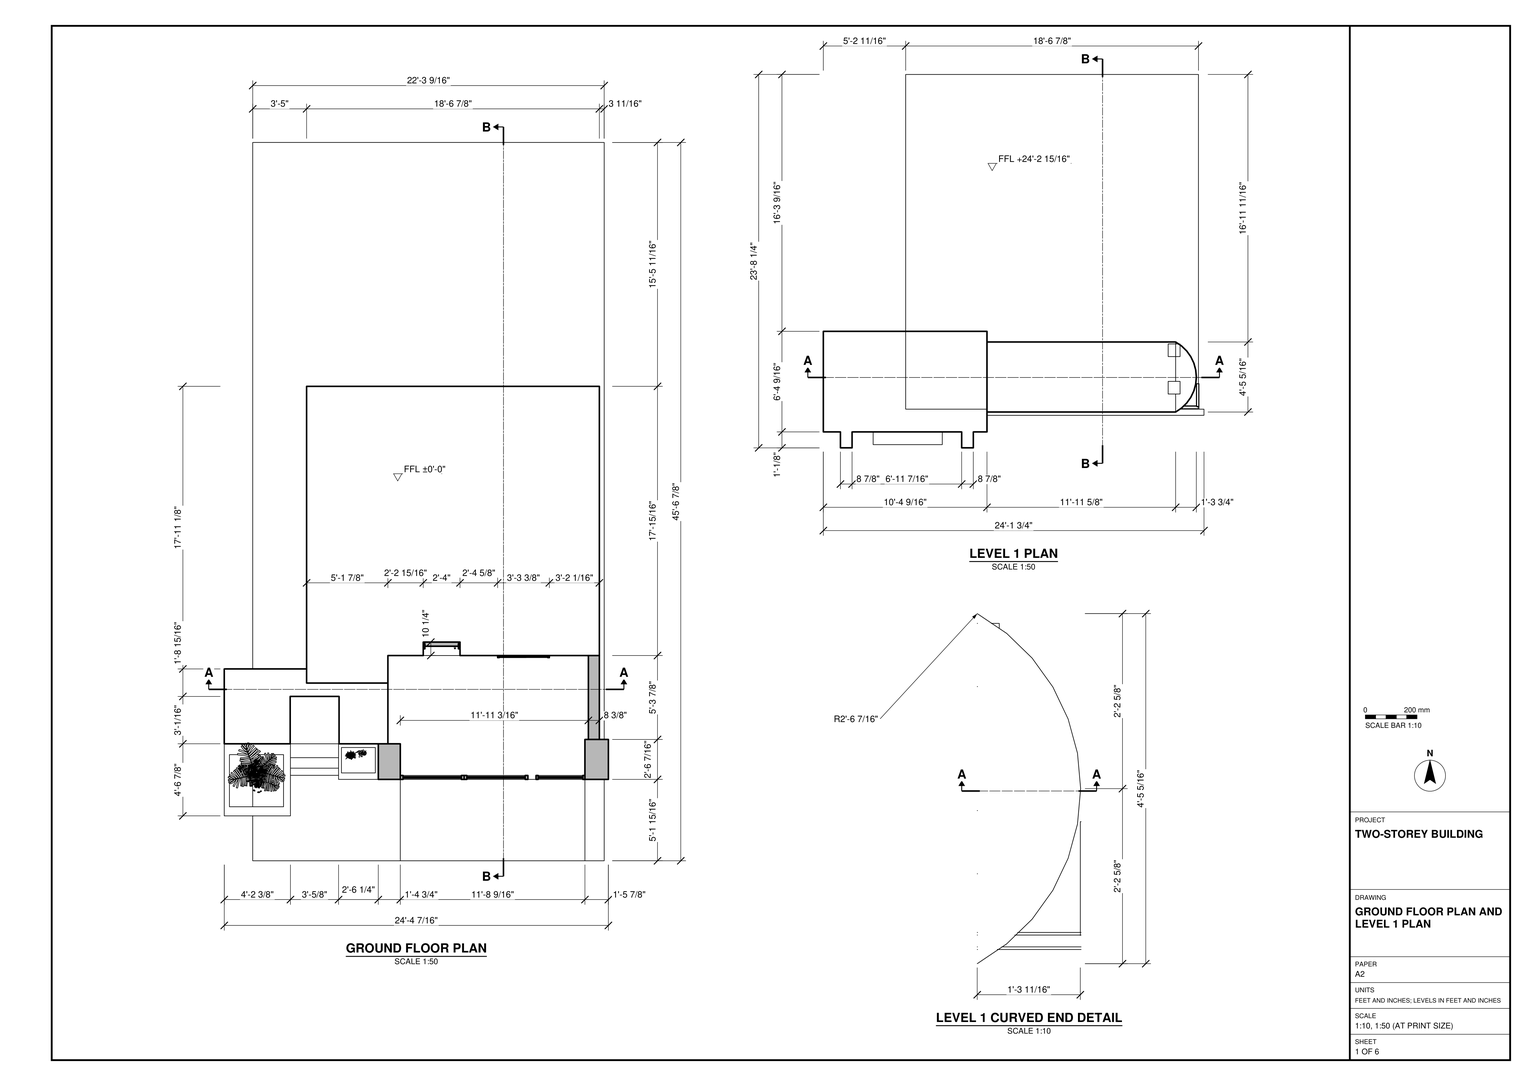
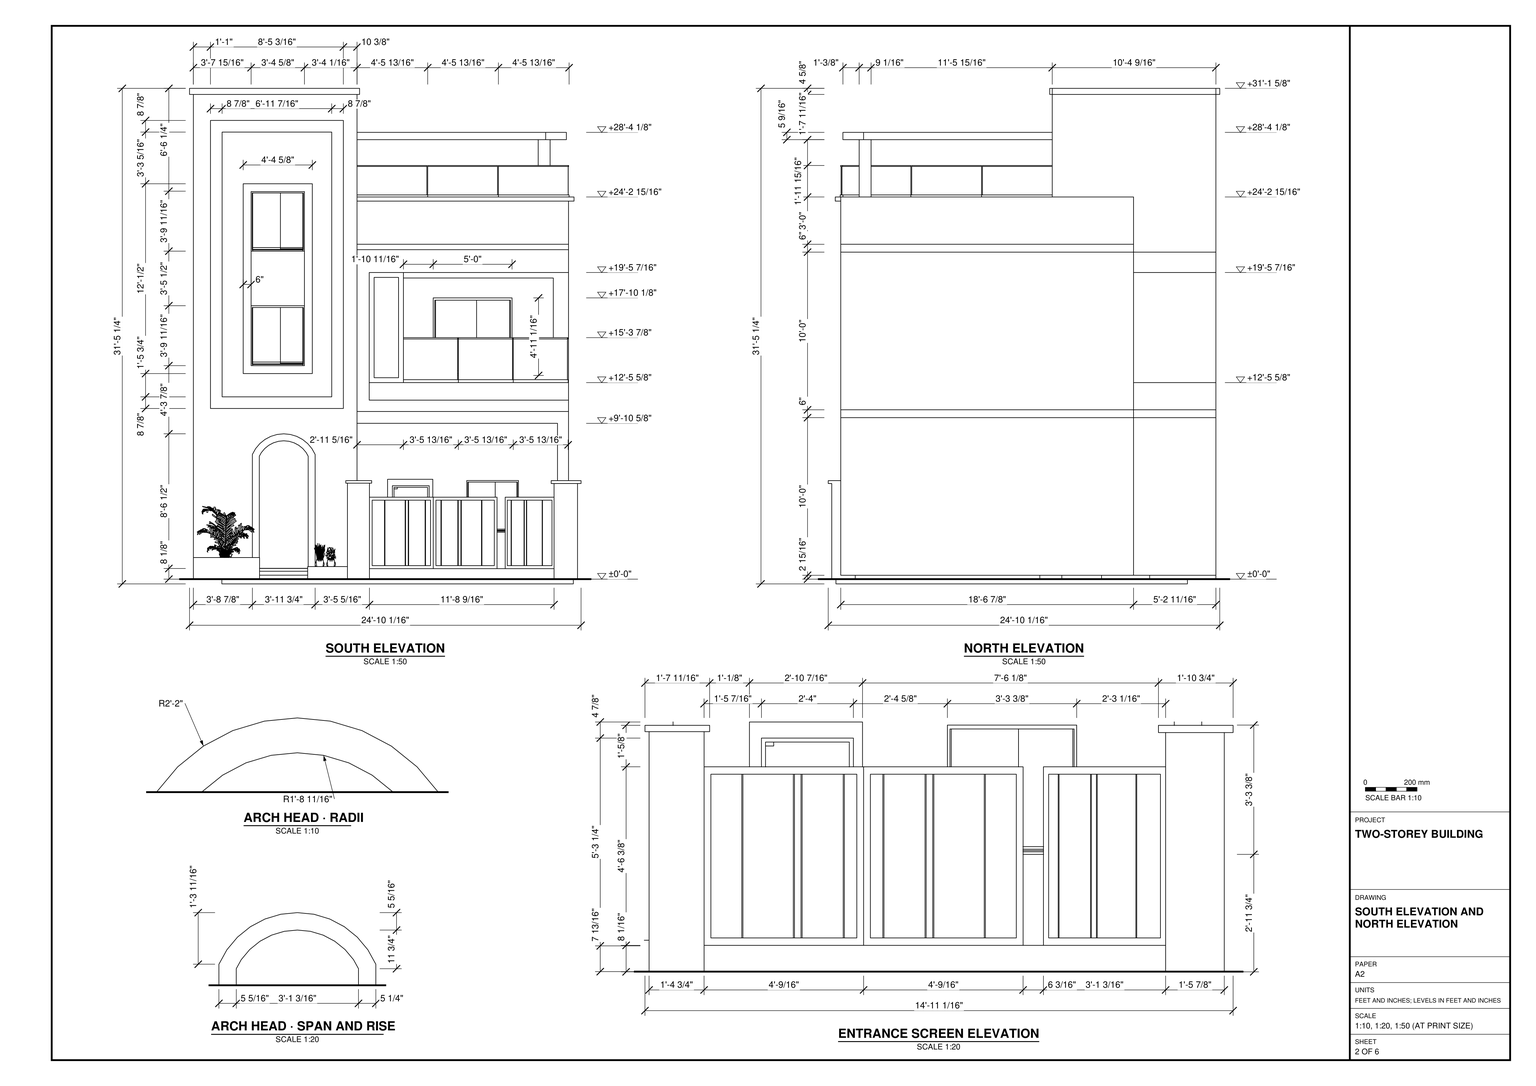
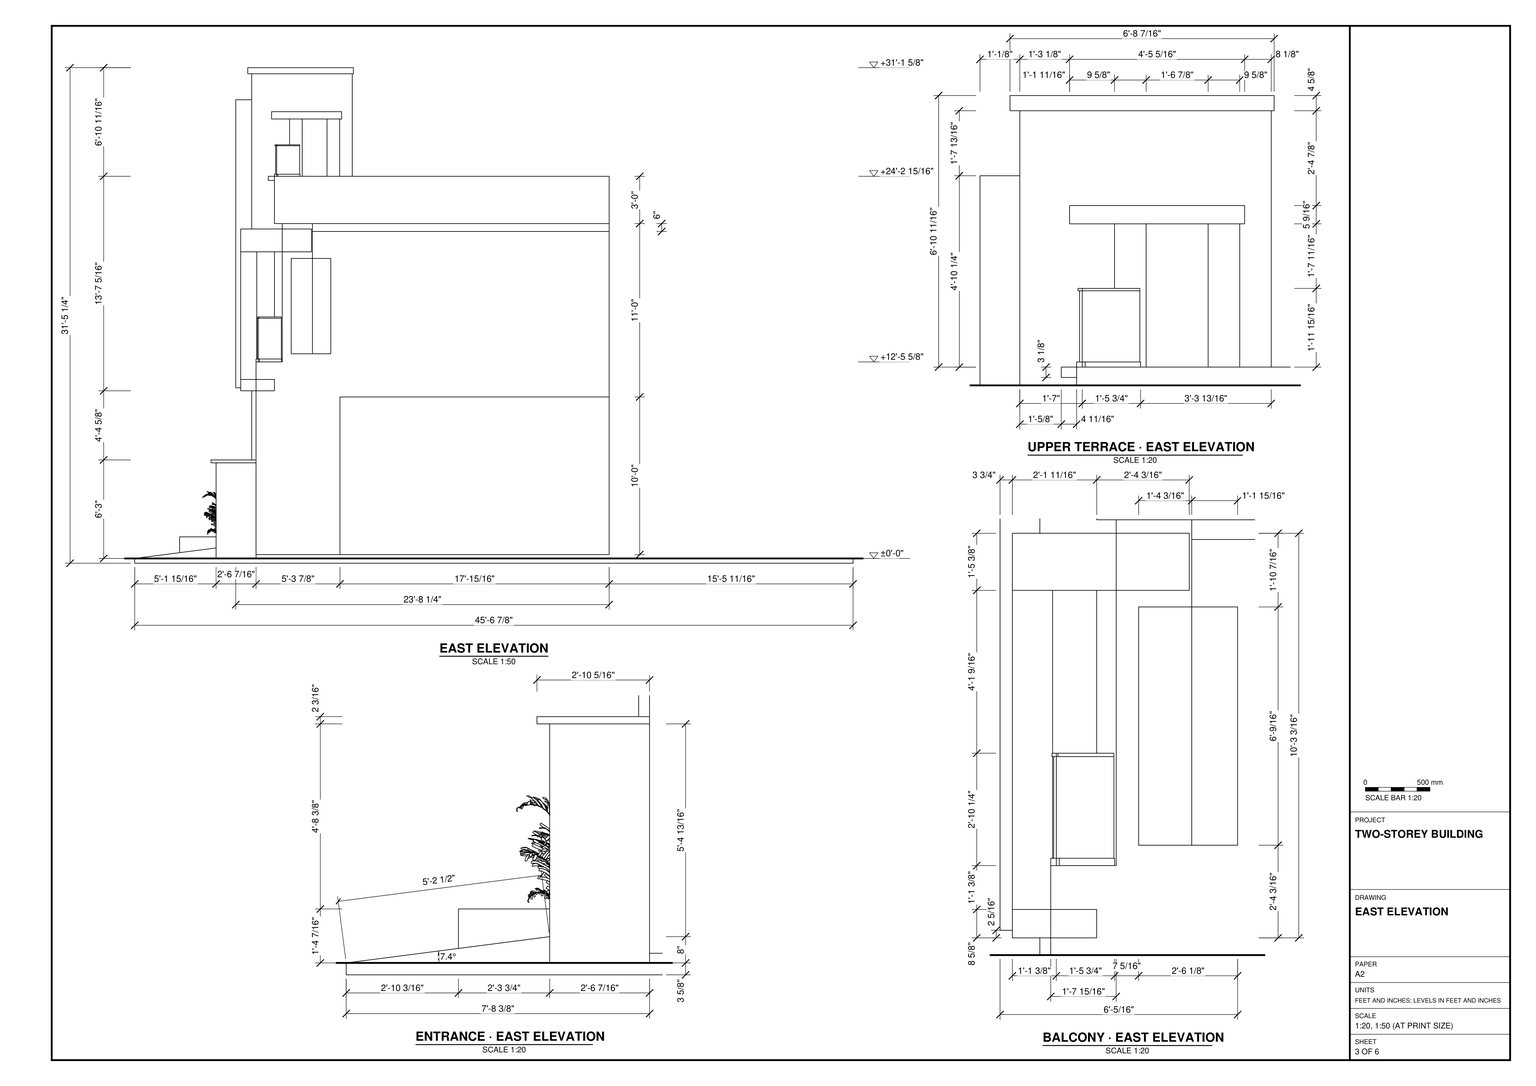
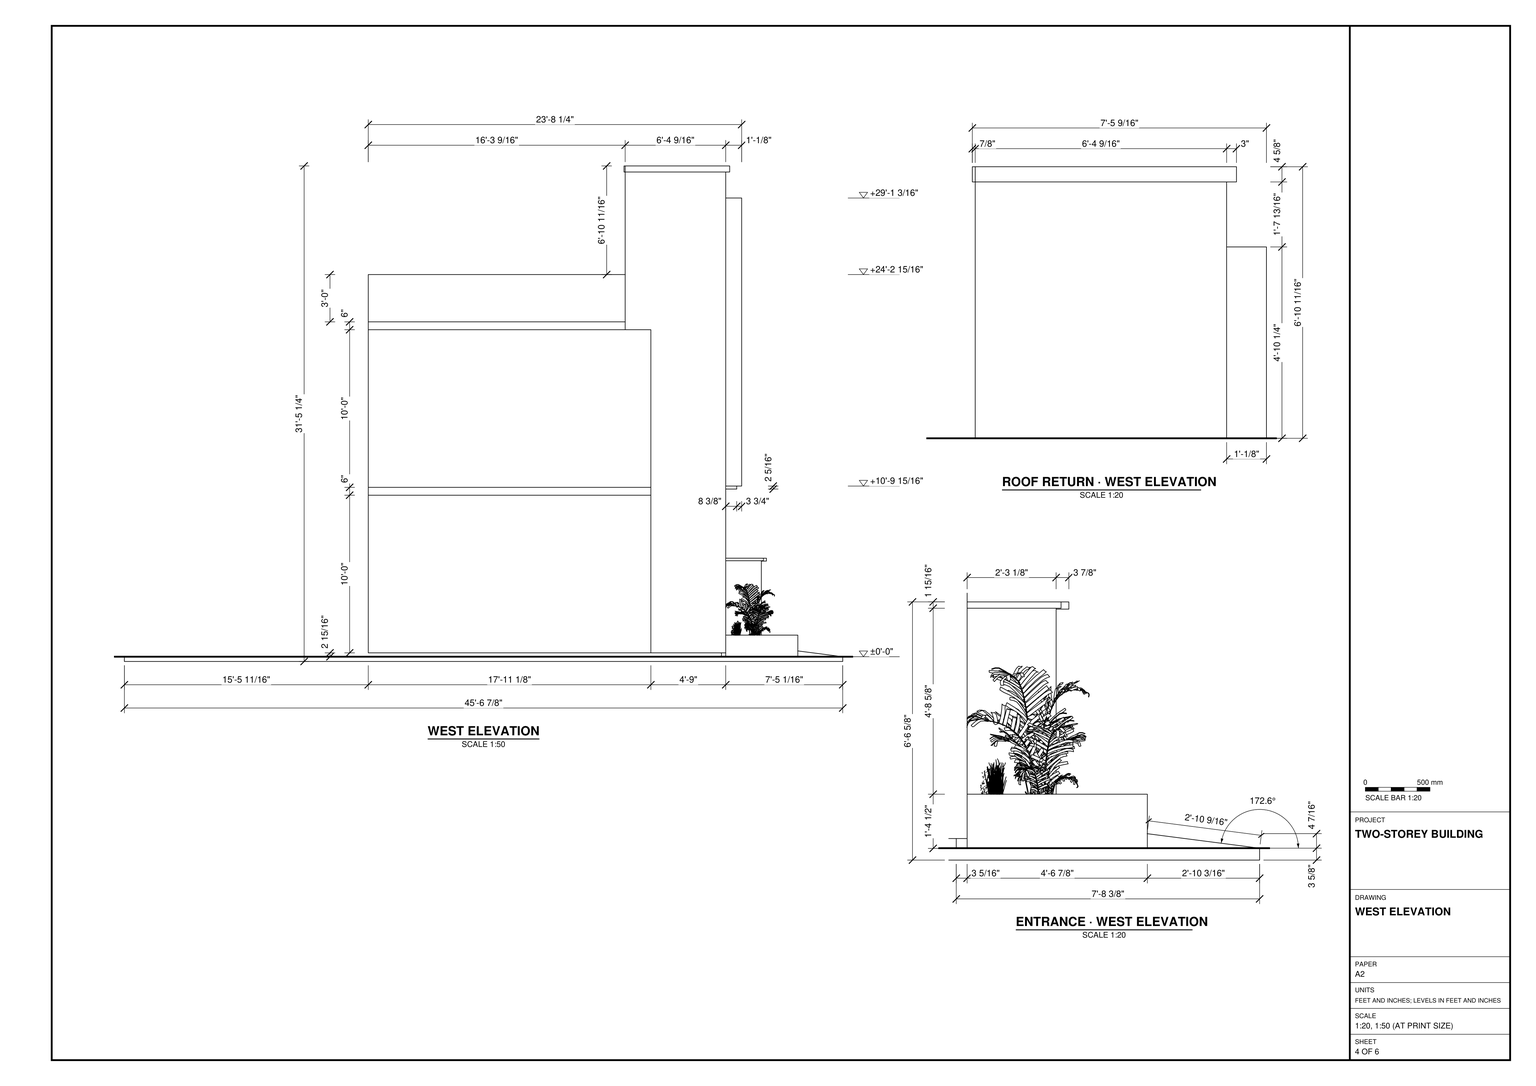
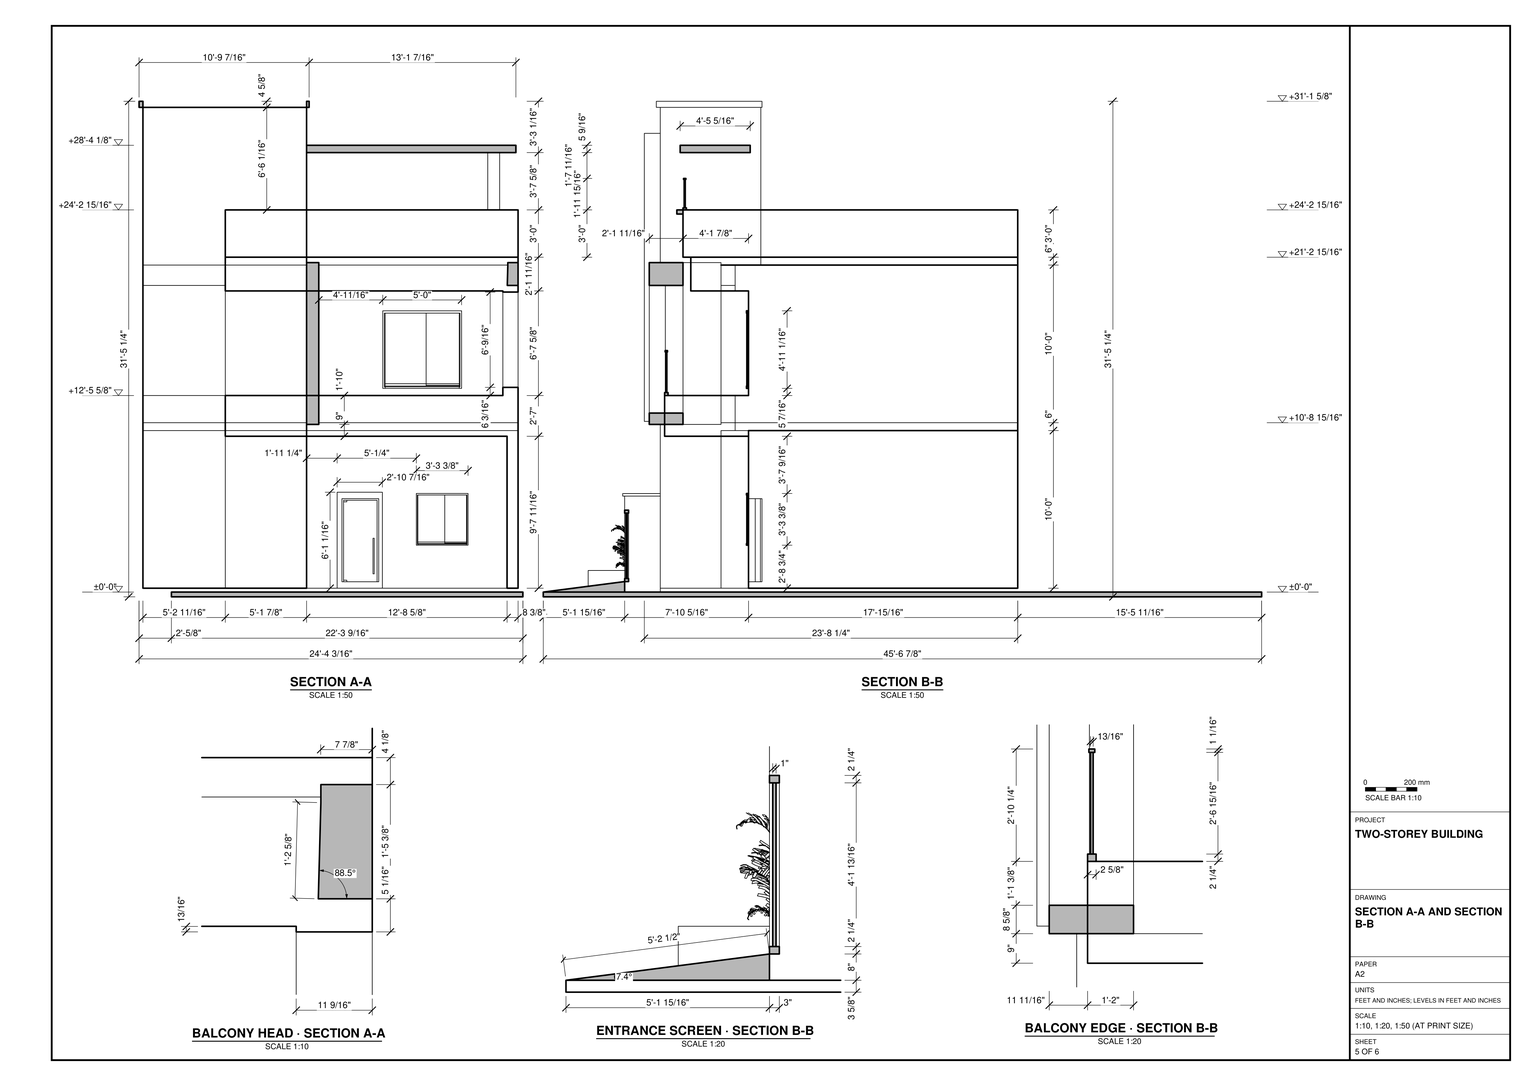
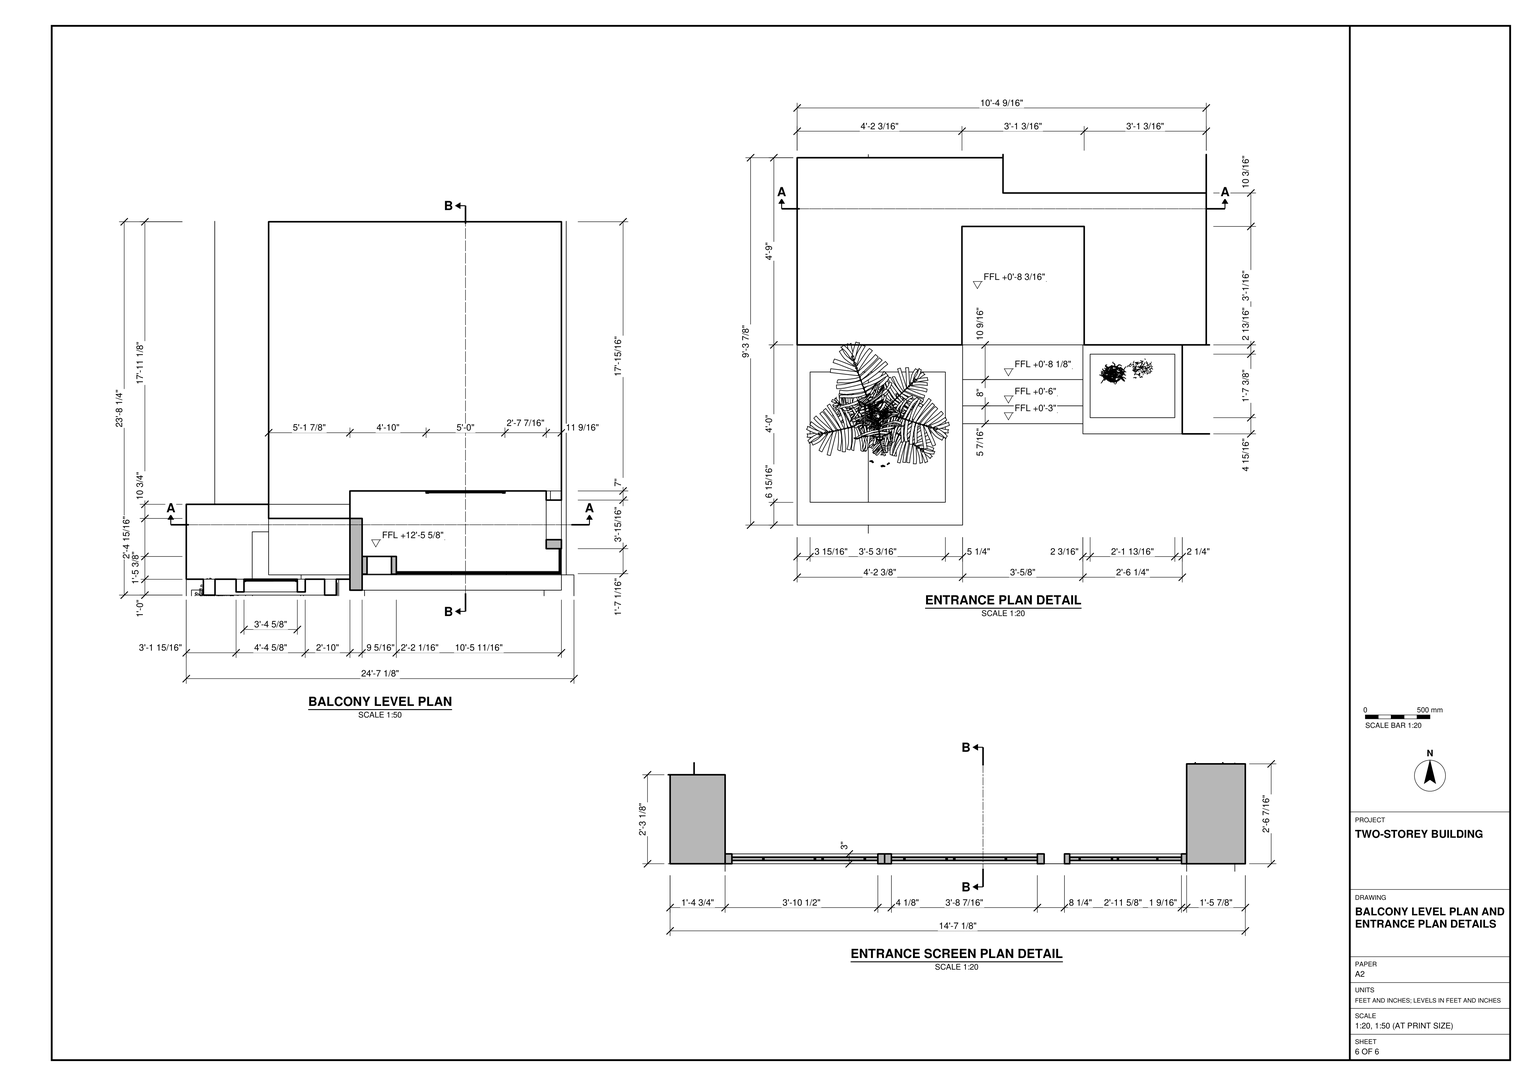
Build the two-storey building in SketchUp using task_files/diagram_01.pdf. Work in feet and inches. The overall model is 24'-10 1/16" wide along X, 45'-6 7/8" deep along Y and 31'-5 1/4" high. Use the ground-floor datum of ±0'-0" and the level marked +24'-2 15/16" on the upper plan.

Lay out the base slab first, leaving the extensions in front of and behind the building as drawn. Follow the plans for the wall positions, thicknesses and offsets, and the elevations for the slab edges, roof profile and openings. On the south face, model the steps and curved head of the entrance beneath the tall framed window bay. Beside it, form the sloping approach and the entrance screen with its vertically divided panels between capped posts. Include the door and window units behind the screen. Above it, recess the balcony behind its outer frame and model its glazing and guard. Use the upper plan and curved-end detail to shape the terrace; include its guard, supports and overhead member beside the taller capped bay.

Place the planting beside the entrance as shown. Decor and loose items such as plants may be any suitable library component. Keep shell elements such as walls, slabs and roof, and each furniture or joinery piece shown, in separate groups or components; use components for repeated parts. Save one SketchUp model as output_files/two_storey_building_arched_entrance_and_roof_terrace.skp.

# SketchUp Ruby script. Lengths in inches.
U = 1.inch
M = Sketchup.active_model
def pt(a) = Geom::Point3d.new(a.map { |v| v * U })
def face(e, loops, mat)
  f = e.add_face(loops[0].map { |a| pt(a) })
  loops[1..].each { |l| e.add_face(l.map { |a| pt(a) }).erase! }
  f.material = f.back_material = mat if mat
  f
end
# faces: each face lists its corners as indices into pts; further lists are holes
def faces(e, pts, list, mat = nil) = list.each { |f| face(e, (f[0].is_a?(Array) ? f : [f]).map { |l| l.map { |i| pts[i] } }, mat) }
# xy, xz, yz: faces in a plane at the given z, y or x. An outline is a flat list of corners, or four numbers for a rectangle; further outlines are holes
def ring(l) = l.size == 4 ? [[l[0], l[1]], [l[2], l[1]], [l[2], l[3]], [l[0], l[3]]] : l.each_slice(2).to_a
def flat(e, list, mat, &to3) = list.each { |f| face(e, (f[0].is_a?(Array) ? f : [f]).map { |l| ring(l).map { |u, v| to3.(u, v) } }, mat) }
def xy(e, z, list, mat = nil) = flat(e, list, mat) { |x, y| [x, y, z] }
def xz(e, y, list, mat = nil) = flat(e, list, mat) { |x, z| [x, y, z] }
def yz(e, x, list, mat = nil) = flat(e, list, mat) { |y, z| [x, y, z] }
def lines(e, pts, list) = list.each { |a, b| e.add_line(pt(pts[a]), pt(pts[b])) }
# prism: a flat outline (further loops are holes) pulled along v
def prism(e, loops, v, mat = nil)
  f = face(e, loops, mat); d = Geom::Vector3d.new(v.map { |x| x * U })
  f.pushpull(f.normal.samedirection?(d) ? d.length : -d.length)
end
def box(e, o, s, mat = nil) = prism(e, [[o, [o[0] + s[0], o[1], o[2]], [o[0] + s[0], o[1] + s[1], o[2]], [o[0], o[1] + s[1], o[2]]]], [0, 0, s[2]], mat)
def at(x, y, z, deg = 0) = Geom::Transformation.translation(pt([x, y, z])) * Geom::Transformation.rotation(ORIGIN, Z_AXIS, deg.degrees)
def axes(o, x, y, z) = Geom::Transformation.new([*x, 0, *y, 0, *z, 0, *pt(o).to_a, 1])
def part(name) = M.definitions.add(name)
# library, detail: a bought-in or finely detailed component or shape, given as its bounding box
def library(name, o, s) = part(name).tap { |d| box(d.entities, o, s) }
def detail(e, o, s) = box(e.add_group.entities, o, s)
def put(e, d, t, mat = nil) = e.add_instance(d, t).tap { |i| i.material = mat if mat }
def group(e, t, mat = nil) = e.add_group.tap { |g| g.transformation = t; g.material = mat if mat }.entities
root = M.entities
M.materials.add("Aluminum_Anodized_Clear\#1").color = [178, 178, 174]
M.materials.add("Aluminum_Anodized_DarkGray\#1").color = [63, 63, 63]
M.materials.add("[0031_PapayaWhip]").color = [255, 239, 213]
M.materials.add("[0134_DimGray]").color = [105, 105, 105]
M.materials.add("[0135_DarkGray]").color = [81, 81, 81]
M.materials.add("[Color M00]").color = [255, 255, 255]
M.materials.add("[Color M03]").color = [170, 170, 170]
M.materials.add("[Color M06]").color = [86, 86, 86]
M.materials.add("[Color M07]").color = [58, 58, 58]
M.materials.add("[Color M08]").color = [30, 30, 30]
M.materials.add("[Granite Tile]").color = [155, 148, 143]
M.materials.add("[Metal_Corrogated_Shiny]").color = [193, 193, 193]
M.materials.add("[Tile Large Brown]").color = [195, 178, 159]
M.materials.add("[Translucent Glass Block Dark]").color = [124, 124, 121]
M.materials["[Translucent Glass Block Dark]"].alpha = 0.8
M.materials.add("[Translucent Glass Gray]").color = [128, 128, 128]
M.materials["[Translucent Glass Gray]"].alpha = 0.5
M.materials.add("[Translucent Glass Sky Reflection]").color = [126, 138, 183]
M.materials["[Translucent Glass Sky Reflection]"].alpha = 0.52
M.materials.add("[Travertine Small Tile]").color = [161, 138, 116]
M.materials.add("[Wood Square Tile 02]").color = [160, 95, 34]
M.materials.add("glass_architectural\#1").color = [217, 197, 188]
M.materials["glass_architectural\#1"].alpha = 0.1
c1 = part("Group\#102")
g1 = group(c1.entities,at(0,0,0))
prism(g1,[[[0,3,72],[70.5,3,72],[70.5,3,0],[0,3,0]],[[67.5,3,3],[67.5,3,69],[3,3,69],[3,3,3]]],[0,-3,0])
c2 = part("Group\#135")
box(c2.entities,[0,0,0],[0.5,1,66])
c3 = part("Group\#148")
box(c3.entities,[0,-1,0],[5.5,1,66])
box(c3.entities,[50.84,-1,0],[13.66,1,66])
box(c3.entities,[28.06,-1,0],[22.28,1,66])
box(c3.entities,[24.66,-1,0],[2.9,1,66])
box(c3.entities,[6,-1,0],[18.16,1,66])
c4 = part("Panelled gate")
g2 = group(c4.entities,at(70.5,0,0),"[Color M08]")
put(g2,c1,axes([70.5,0,0],[-1,0,0],[0,1,0],[0,0,1]))
g3 = group(g2,at(3,2,3))
g4 = group(g3,at(0,-1,0))
box(g4,[0,0,0],[5.5,1,66])
box(g4,[50.84,0,0],[13.66,1,66])
box(g4,[28.06,0,0],[22.28,1,66])
box(g4,[24.66,0,0],[2.9,1,66])
box(g4,[6,0,0],[18.16,1,66])
put(g3,c2,axes([50.34,0,0],[1,0,0],[0,-1,0],[0,0,1]))
put(g3,c2,axes([24.16,0,0],[1,0,0],[0,-1,0],[0,0,1]))
put(g3,c2,axes([27.56,0,0],[1,0,0],[0,-1,0],[0,0,1]))
put(g3,c2,axes([5.5,0,0],[1,0,0],[0,-1,0],[0,0,1]))
g5 = group(c4.entities,at(70.5,0,0),"[Color M08]")
put(g5,c1,at(-70.5,0,0))
g6 = group(g5,at(-3,2,3,-180))
put(g6,c3,at(0,1,0))
put(g6,c2,at(50.34,0,0))
put(g6,c2,at(24.16,0,0))
put(g6,c2,at(27.56,0,0))
put(g6,c2,at(5.5,0,0))
g7 = group(c4.entities,at(150,0,0),"[Color M08]")
put(g7,c1,axes([54,0,0],[-0.76596,0,0],[0,1,0],[0,0,1]))
g8 = group(g7,at(2.3,2,3))
put(g8,c3,axes([0,-1,0],[0.76596,0,0],[0,-1,0],[0,0,1]))
put(g8,c2,axes([38.55,0,0],[0.76596,0,0],[0,-1,0],[0,0,1]))
put(g8,c2,axes([18.5,0,0],[0.76596,0,0],[0,-1,0],[0,0,1]))
put(g8,c2,axes([21.11,0,0],[0.76596,0,0],[0,-1,0],[0,0,1]))
put(g8,c2,axes([4.22,0,0],[0.76596,0,0],[0,-1,0],[0,0,1]))
c5 = part("Component\#1")
box(c5.entities,[0,0,0],[0.31,1.57,3.15],"[Metal_Corrogated_Shiny]")
c6 = part("Door pull handle")
prism(c6.entities,[[[0,1.18,35.04],[0,1.18,35.43],[1.97,1.18,35.43],[1.97,1.18,0],[0,1.18,0],[0,1.18,0.39],[1.57,1.18,0.39],[1.57,1.18,35.04]]],[0,-1.18,0],"[Color M07]")
c7 = part("Framed door")
g9 = group(c7.entities,at(1.61,1.57,0))
g10 = group(g9,at(-1.8125,0,0))
g11 = group(g10,at(1.77,0,0))
p = [[0.59,0,81.1],[0.59,32.28,81.1]]
lines(g11,p,[[0,1]])
g12 = group(g11,at(0.59,0,0))
yz(g12,0,[[0,0,32.28,81.1]],"[Translucent Glass Gray]")
g13 = group(g10,at(-1.9,0,0))
put(g13,c5,axes([4.11,0,81.1],[1,0,0],[0,0,-1],[0,1,0]))
put(g13,c5,axes([4.11,0,1.57],[1,0,0],[0,0,-1],[0,1,0]))
g14 = group(g10,at(0,28.35,7.875))
put(g14,c6,axes([2.36,0,0],[-1,0,0],[0,1,0],[0,0,1]))
put(g14,c6,at(2.36,0,0))
g15 = group(c7.entities,at(4.13,0,0))
g16 = group(g15,at(-3.9375,0,0))
prism(g16,[[[3.9375,33.86,0],[3.9375,35.43,0],[3.9375,35.43,82.68],[3.9375,0,82.68],[3.9375,0,0],[3.9375,1.57,0],[3.9375,1.57,81.1],[3.9375,33.86,81.1]]],[-3.9375,0,0],"[Metal_Corrogated_Shiny]")
c8 = part("door2")
put(c8.entities,c7,at(0,4.13,0,-90))
c9 = part("Agrupar\#2")
xy(c9.entities,0,[[0,0,1.57,39.37]])
xy(c9.entities,0.79,[[0.2,0.79,0.34,38.58],[0.34,0.79,0.49,38.58],[1.23,0.79,1.38,38.58]])
xy(c9.entities,1.18,[[0.08,0.79,0.2,0.79,0.2,38.58,0.08,38.58,0.08,38.1875,0,38.1875,0,1.18,0.08,1.18],[0.49,0.79,0.61,17.72],[0.67,0.79,0.79,17.72],[0.79,0.79,0.94,38.58],[1.38,0.79,1.5,0.79,1.5,1.18,1.57,1.18,1.57,38.1875,1.5,38.1875,1.5,38.58,1.38,38.58],
  [0.94,21.65,1.06,38.58],[1.11,21.65,1.23,38.58]])
xy(c9.entities,1.57,[[0.61,0.79,0.67,17.72],[1.06,21.65,1.11,38.58]])
xy(c9.entities,2.36,[[0.94,0.79,0.99,21.65],[0.99,0.79,1.17,0.84],[1.17,0.79,1.23,21.65],[0.49,17.72,0.54,38.58],[0.74,17.72,0.79,38.58],
  [0.54,38.54,0.74,38.58]])
xy(c9.entities,38.1875,[[0.08,0.79,0.08,1.18,0,1.18,0,38.1875,0.08,38.1875,0.08,38.58,0.49,38.58,0.49,0.79],[0.79,0.79,0.94,38.58],[1.23,0.79,1.23,38.58,1.5,38.58,1.5,38.1875,1.57,38.1875,1.57,1.18,1.5,1.18,1.5,0.79]])
xy(c9.entities,38.58,[[[0.49,0.79,0.79,38.58],[0.54,17.72,0.74,38.54]],[0.94,0.79,1.23,38.58]])
xy(c9.entities,38.98,[[0.99,0.84,1.17,21.65]])
xy(c9.entities,39.37,[[0,0,1.57,39.37]])
xz(c9.entities,0,[[0,0,1.57,39.37]])
xz(c9.entities,0.79,[[0.2,0.79,0.2,1.18,0.08,1.18,0.08,38.1875,0.49,38.1875,0.49,38.58,0.79,38.58,0.79,38.1875,0.94,38.1875,0.94,38.58,1.23,38.58,1.23,38.1875,1.5,38.1875,1.5,1.18,1.38,1.18,1.38,0.79,1.23,0.79,1.23,2.36,0.94,2.36,0.94,1.18,0.67,1.18,0.67,1.57,0.61,1.57,0.61,1.18,0.49,1.18,0.49,0.79]])
xz(c9.entities,0.84,[[0.99,2.36,1.17,38.98]])
xz(c9.entities,1.18,[[0,1.18,0.08,38.1875],[1.5,1.18,1.57,38.1875]])
xz(c9.entities,17.72,[[0.49,1.18,0.61,1.18,0.61,1.57,0.67,1.57,0.67,1.18,0.79,1.18,0.79,2.36,0.74,2.36,0.74,38.58,0.54,38.58,0.54,2.36,0.49,2.36]],"[Translucent Glass Gray]")
xz(c9.entities,21.65,[[0.94,1.18,0.94,2.36,0.99,2.36,0.99,38.98,1.17,38.98,1.17,2.36,1.23,2.36,1.23,1.18,1.11,1.18,1.11,1.57,1.06,1.57,1.06,1.18]],"[Translucent Glass Gray]")
xz(c9.entities,38.1875,[[0,1.18,0.08,38.1875],[1.5,1.18,1.57,38.1875]])
xz(c9.entities,38.54,[[0.54,2.36,0.74,38.58]])
xz(c9.entities,38.58,[[0.2,0.79,0.49,0.79,0.49,2.36,0.79,2.36,0.79,1.18,1.06,1.18,1.06,1.57,1.11,1.57,1.11,1.18,1.23,1.18,1.23,0.79,1.38,0.79,1.38,1.18,1.5,1.18,1.5,38.1875,1.23,38.1875,1.23,38.58,0.94,38.58,0.94,38.1875,0.79,38.1875,0.79,38.58,0.49,38.58,0.49,38.1875,0.08,38.1875,0.08,1.18,0.2,1.18]])
xz(c9.entities,39.37,[[0,0,1.57,39.37]])
yz(c9.entities,0,[[[0,0,39.37,39.37],[1.18,1.18,38.1875,38.1875]]],"[Color M00]")
yz(c9.entities,0.08,[[0.79,1.18,1.18,38.1875],[38.1875,1.18,38.58,38.1875]])
yz(c9.entities,0.2,[[0.79,0.79,38.58,1.18]])
yz(c9.entities,0.49,[[0.79,0.79,17.72,1.18],[17.72,0.79,38.58,2.36],[0.79,38.1875,38.58,38.58]])
yz(c9.entities,0.54,[[17.72,2.36,38.54,38.58]],"[Translucent Glass Gray]")
yz(c9.entities,0.61,[[0.79,1.18,17.72,1.57]])
yz(c9.entities,0.67,[[0.79,1.18,17.72,1.57]])
yz(c9.entities,0.74,[[17.72,2.36,38.54,38.58]],"[Translucent Glass Gray]")
yz(c9.entities,0.79,[[17.72,1.18,38.58,2.36],[0.79,38.1875,38.58,38.58]])
yz(c9.entities,0.94,[[0.79,1.18,21.65,2.36],[0.79,38.1875,38.58,38.58]])
yz(c9.entities,0.99,[[0.84,2.36,21.65,38.98]],"[Translucent Glass Gray]")
yz(c9.entities,1.06,[[21.65,1.18,38.58,1.57]])
yz(c9.entities,1.11,[[21.65,1.18,38.58,1.57]])
yz(c9.entities,1.17,[[0.84,2.36,21.65,38.98]],"[Translucent Glass Gray]")
yz(c9.entities,1.23,[[0.79,0.79,21.65,2.36],[21.65,0.79,38.58,1.18],[0.79,38.1875,38.58,38.58]])
yz(c9.entities,1.38,[[0.79,0.79,38.58,1.18]])
yz(c9.entities,1.5,[[0.79,1.18,1.18,38.1875],[38.1875,1.18,38.58,38.1875]])
yz(c9.entities,1.57,[[0,0,1.18,0,1.18,38.1875,38.1875,38.1875,38.1875,0,39.37,0,39.37,39.37,0,39.37],[1.18,0,38.1875,1.18]])
c10 = part("GLASS")
box(c10.entities,[0,0,0],[48,0.8,36])
c11 = part("STEEL BAR")
box(c11.entities,[0,-0.1,0],[48,1.8,1.2])
c12 = part("LOWER PART")
box(c12.entities,[0,-0.6,0],[48.6,2.6,2.6])
c13 = part("BALCONY GLASS ")
put(c13.entities,c10,at(0,0.9,2.6),"glass_architectural\#1")
put(c13.entities,c11,at(0,0.5,38.6),"Aluminum_Anodized_DarkGray\#1")
put(c13.entities,c12,at(0,0.6,0),"Aluminum_Anodized_Clear\#1")
c14 = part("NO 3")
put(c14.entities,c13,at(0,0,0))
put(c14.entities,c13,at(48.6,0,0))
put(c14.entities,c13,at(97.2,0,0))
c15 = library("trol",[-1.07,-0.37,0],[9.56,15.9,13.04])
c16 = library("KentiaPalm",[-22.86,-14.31,0],[47.49,43.96,59.125])
box(root,[265.44,117.91,291],[9.06,9.62,44.5625])
xy(root,0,[[2.9375,34.1875,53.33,89.07],[277.5,61.96,295.36,92.375]])
xy(root,0.0625,[[136.96,0,277.5,61.96],[6.88,41.13,48.07,80.81],[89.95,61.96,120.21,89.07],[120.21,61.96,136.96,89.07],[53.33,65.07,89.95,70.5],
  [53.33,70.5,89.95,78.5],[53.33,78.5,89.95,89.07]])
xy(root,1.25,[[92.15,66.89,117.95,86.24]])
xy(root,3.0625,[[53.33,65.07,89.95,70.5]],"[Travertine Small Tile]")
xy(root,6.0625,[[53.33,70.5,89.95,78.5]],"[Travertine Small Tile]")
xy(root,8.1875,[[53.33,78.5,89.95,89.07]],"[Travertine Small Tile]")
xy(root,9.625,[[[89.95,61.96,120.21,89.07],[92.15,66.89,117.95,86.24]]],"[Travertine Small Tile]")
xy(root,16.5,[[[2.9375,34.1875,53.33,89.07],[6.88,41.13,48.07,80.81]]],"[Travertine Small Tile]")
xy(root,72.86,[[275.32,58.09,298.05,61.96],[275.32,61.96,277.5,92.375],[295.36,61.96,298.05,92.375]])
xy(root,73.14,[[118.96,60.46,136.96,61.96],[136.96,60.46,138.65,89.07],[118.96,61.96,120.21,89.07]])
xy(root,75.0625,[[275.32,58.09,298.05,92.375],[118.96,60.46,138.65,89.07]],"[Travertine Small Tile]")
xy(root,127.6875,[[127.51,80.69,127.51,135.3125,136.8,135.3125,136.8,106.375,288.5,106.375,288.5,80.69]])
xy(root,136.33,[[136.8,80.69,288.5,106.375]])
xy(root,149.6875,[[136.8,92.9375,162.84,106.375]])
xy(root,153.41,[[140.52,92.9375,159.12,106.375]])
xy(root,229.78,[[140.52,92.9375,159.12,106.375]])
xy(root,233.5,[[136.8,80.69,136.8,92.9375,162.84,92.9375,162.84,106.375,280.29,106.375,280.29,134.5625,288.5,134.5625,288.5,80.69],[136.8,92.9375,162.84,106.375]])
xy(root,250.89,[[127.51,80.69,288.5,80.69,288.5,134.5625,280.68,134.5625,280.68,106.375,136.8,106.375,136.8,135.3125,127.51,135.3125]])
xy(root,287.84,[[127.51,101.6875,292.69,106.375]],"[Color M06]")
xy(root,291,[[265.44,146.41,274.5,156.03]])
xy(root,291,[[127.51,101.6875,292.69,106.375]],"[Color M06]")
xy(root,334.625,[[127.51,104.21,127.51,157.53,271.14,157.53,271.14,156.03,265.44,156.03,265.44,146.41,271.14,146.41,271.14,104.21],[271.14,104.21,271.14,146.41,274.5,146.41,274.5,155.26,275.62,154.51,279.5,150.74,282.66,146.35,284.98,141.47,286.41,136.26,286.89,130.87,286.41,125.49,284.98,120.27,282.66,115.39,279.5,111,275.62,107.23],[265.44,146.41,271.14,156.03],[271.14,146.41,274.5,146.41,274.5,155.26,273.36,156.03,271.14,156.03],[274.5,155.26,274.5,156.03,273.36,156.03],
  [271.14,156.03,271.14,157.53,273.36,156.03]])
xy(root,340.1875,[[127.51,104.21,271.14,104.21,275.62,107.23,279.5,111,282.66,115.39,284.98,120.27,286.41,125.49,286.89,130.87,286.41,136.26,284.98,141.47,282.66,146.35,279.5,150.74,275.62,154.51,271.14,157.53,127.51,157.53]])
xy(root,369.07,[[0,86.07,0,165.625,2.9375,165.625,2.9375,89.07,127.51,89.07,127.51,166.5,129.45,166.5,129.45,86.07]])
xy(root,373.69,[[0,86.07,129.45,86.07,129.45,166.5,127.51,166.5,127.51,89.07,2.9375,89.07,2.9375,165.625,0,165.625]])
xz(root,34.1875,[[2.9375,0,53.33,16.5]],"[Travertine Small Tile]")
xz(root,41.13,[[6.88,0.0625,48.07,16.5]])
xz(root,58.09,[[275.32,72.86,298.05,75.0625]])
xz(root,60.46,[[118.96,73.14,138.65,75.0625]])
xz(root,61.96,[[136.96,0.0625,277.5,8.0625]])
xz(root,61.96,[[277.5,0,295.36,72.86],[89.95,0.0625,120.21,9.625],[120.21,0.0625,136.96,73.14]],"[Travertine Small Tile]")
xz(root,65.07,[[53.33,0.0625,89.95,3.0625]],"[Travertine Small Tile]")
xz(root,66.89,[[92.15,1.25,117.95,9.625]])
xz(root,70.5,[[53.33,0.0625,89.95,3.0625]])
xz(root,70.5,[[53.33,3.0625,89.95,6.0625]],"[Travertine Small Tile]")
xz(root,78.5,[[53.33,0.0625,89.95,6.0625]])
xz(root,78.5,[[53.33,6.0625,89.95,8.1875]],"[Travertine Small Tile]")
xz(root,80.69,[[127.51,127.6875,288.5,127.6875,288.5,136.33,136.8,136.33,136.8,233.5,288.5,233.5,288.5,250.89,127.51,250.89]])
xz(root,80.81,[[6.88,0.0625,48.07,16.5]])
xz(root,86.07,[[0,369.07,129.45,373.69]],"[0134_DimGray]")
xz(root,86.24,[[92.15,1.25,117.95,9.625]])
xz(root,89.07,[[2.9375,0,53.33,16.5],[53.33,0.0625,89.95,8.1875],[89.95,0.0625,120.21,9.625],[120.21,0.0625,120.21,73.14,118.96,73.14,118.96,75.0625,138.65,75.0625,138.65,73.14,136.96,73.14,136.96,0.0625],[2.9375,369.07,127.51,373.69]])
xz(root,92.375,[[277.5,0,277.5,72.86,275.32,72.86,275.32,75.0625,298.05,75.0625,298.05,72.86,295.36,72.86,295.36,0]])
xz(root,92.9375,[[[136.8,149.6875,162.84,233.5],[140.52,153.41,159.12,229.78]]])
xz(root,101.6875,[[127.51,287.84,292.69,291]],"[Color M06]")
xz(root,104.21,[[127.51,334.625,271.14,340.1875]])
xz(root,106.375,[[136.8,127.6875,288.5,136.33],[[136.8,149.6875,162.84,233.5],[140.52,153.41,159.12,229.78]],[136.8,233.5,280.29,250.89],[280.29,233.5,280.29,250.89,280.68,250.89,280.68,248.14],[127.51,287.84,292.69,291]])
xz(root,106.375,[[140.52,153.41,159.12,229.78]],"[Translucent Glass Block Dark]")
xz(root,134.5625,[[280.29,233.5,280.68,248.14,280.68,250.89,288.5,250.89,288.5,233.5]])
xz(root,135.3125,[[127.51,127.6875,136.8,250.89]])
xz(root,146.41,[[265.44,291,274.5,334.625]])
xz(root,156.03,[[265.44,291,274.5,334.625]])
xz(root,157.53,[[127.51,334.625,271.14,340.1875]])
xz(root,165.625,[[0,369.07,2.9375,373.69]])
xz(root,166.5,[[127.51,369.07,129.45,373.69]])
yz(root,0,[[86.07,369.07,165.625,373.69]],"[0134_DimGray]")
yz(root,2.9375,[[89.07,369.07,165.625,373.69]])
yz(root,2.9375,[[34.1875,0,89.07,16.5]],"[Travertine Small Tile]")
yz(root,6.88,[[41.13,0.0625,80.81,16.5]])
yz(root,48.07,[[41.13,0.0625,80.81,16.5]])
yz(root,53.33,[[65.07,0.0625,70.5,3.0625],[70.5,0.0625,78.5,6.0625],[78.5,0.0625,89.07,8.1875]])
yz(root,53.33,[[34.1875,0,89.07,0,89.07,0.0625,65.07,0.0625,65.07,3.0625,70.5,3.0625,70.5,6.0625,78.5,6.0625,78.5,8.1875,89.07,8.1875,89.07,16.5,34.1875,16.5]],"[Travertine Small Tile]")
yz(root,89.95,[[61.96,0.0625,65.07,3.0625],[65.07,0.0625,70.5,3.0625],[70.5,0.0625,78.5,6.0625],[78.5,0.0625,89.07,8.1875]])
yz(root,89.95,[[61.96,3.0625,61.96,9.625,89.07,9.625,89.07,8.1875,78.5,8.1875,78.5,6.0625,70.5,6.0625,70.5,3.0625]],"[Travertine Small Tile]")
yz(root,92.15,[[66.89,1.25,86.24,9.625]])
yz(root,117.95,[[66.89,1.25,86.24,9.625]])
yz(root,118.96,[[60.46,73.14,89.07,75.0625]])
yz(root,120.21,[[61.96,0.0625,89.07,9.625]])
yz(root,120.21,[[61.96,9.625,89.07,73.14]],"[Travertine Small Tile]")
yz(root,127.51,[[80.69,127.6875,135.3125,250.89],[101.6875,287.84,106.375,291],[104.21,334.625,157.53,340.1875],[89.07,369.07,166.5,373.69]])
yz(root,129.45,[[86.07,369.07,166.5,373.69]],"[0134_DimGray]")
yz(root,136.8,[[106.375,127.6875,135.3125,127.6875,135.3125,250.89,106.375,250.89,106.375,233.5,92.9375,233.5,92.9375,149.6875,106.375,149.6875],[80.69,136.33,106.375,136.33,106.375,149.6875,92.9375,149.6875,92.9375,233.5,80.69,233.5]])
yz(root,136.96,[[0,0.0625,61.96,8.0625,61.96,0.0625]])
yz(root,136.96,[[61.96,0.0625,89.07,73.14]],"[Travertine Small Tile]")
yz(root,138.65,[[60.46,73.14,89.07,75.0625]])
yz(root,140.52,[[92.9375,153.41,106.375,229.78]])
yz(root,159.12,[[92.9375,153.41,106.375,229.78]])
yz(root,162.84,[[92.9375,149.6875,106.375,233.5]])
yz(root,265.44,[[146.41,291,156.03,334.625]])
yz(root,274.5,[[146.41,291,156.03,334.625]])
yz(root,275.32,[[58.09,72.86,92.375,75.0625]])
yz(root,277.5,[[61.96,0,92.375,72.86],[0,0.0625,61.96,0.0625,61.96,8.0625]])
yz(root,280.68,[[106.375,248.14,134.5625,250.89]])
yz(root,288.5,[[80.69,127.6875,106.375,136.33],[80.69,233.5,134.5625,250.89]])
yz(root,292.69,[[101.6875,287.84,106.375,291]],"[Color M06]")
yz(root,295.36,[[61.96,0,92.375,72.86]],"[Travertine Small Tile]")
yz(root,298.05,[[58.09,72.86,92.375,75.0625]])
p = [[136.96,61.96,8.0625],[136.96,0,0.0625],[277.5,0,0.0625],[277.5,61.96,8.0625],[280.29,106.375,233.5],[280.68,106.375,248.14],
  [280.68,134.5625,248.14],[280.29,134.5625,233.5],[275.62,107.23,340.1875],[271.14,104.21,340.1875],[271.14,104.21,334.625],[275.62,107.23,334.625],
  [279.5,111,340.1875],[279.5,111,334.625],[282.66,115.39,340.1875],[282.66,115.39,334.625],[284.98,120.27,340.1875],[284.98,120.27,334.625],
  [286.41,125.49,340.1875],[286.41,125.49,334.625],[286.89,130.87,340.1875],[286.89,130.87,334.625],[286.41,136.26,340.1875],[286.41,136.26,334.625],
  [284.98,141.47,340.1875],[284.98,141.47,334.625],[282.66,146.35,340.1875],[282.66,146.35,334.625],[279.5,150.74,340.1875],[279.5,150.74,334.625],
  [275.62,154.51,340.1875],[275.62,154.51,334.625],[271.14,157.53,340.1875],[274.5,155.26,334.625],[273.36,156.03,334.625],[271.14,157.53,334.625],
  [280.69,106.375,248.61],[46.87,89.07,249.75],[87.48,89.07,249.75],[46.87,89.07,205.33],[87.48,89.07,205.33]]
faces(root,p,[[0,1,2,3]],"[Tile Large Brown]")
faces(root,p,[[4,5,6,7],[8,9,10,11],[12,8,11,13],[14,12,13,15],[16,14,15,17],[18,16,17,19],[20,18,19,21],[22,20,21,23],
  [24,22,23,25],[26,24,25,27],[28,26,27,29],[30,28,29,31],[32,30,31,33,34,35]])
lines(root,p,[[5,36],[37,38],[39,40]])
put(root,c4,axes([136.96,61.96,8.0625],[0.68893,0,0],[0,1,0],[0,0,0.7552]))
put(root,c8,axes([154.42,161.375,7.91],[0.79023,0,0],[0,1,0],[0,0,0.76529]),"[Translucent Glass Sky Reflection]")
put(root,c9,at(211.05,156.25,35.77,-90),"[Translucent Glass Sky Reflection]")
put(root,c9,axes([185.52,156.25,155.13],[0,-1,0],[1.524,0,0],[0,0,1.5]),"[Translucent Glass Sky Reflection]")
put(root,c14,axes([162.84,92.375,149.6875],[0.86,0,0],[0,1,0],[0,0,0.86]))
put(root,c13,axes([288.23,94.08,149.6875],[0,0.36547,0],[-0.63,0,0],[0,0,0.86]))
put(root,c14,axes([127.51,106.375,291],[1.10725,0,0],[0,1,0],[0,0,0.602]))
put(root,c13,axes([288.95,108.08,291],[0,0.36547,0],[-0.81113,0,0],[0,0,0.602]))
put(root,c9,axes([46.87,89.07,249.75],[0,-1,0],[1.03151,0,0],[0,0,1.15984]),"[Translucent Glass Sky Reflection]")
put(root,c9,axes([46.87,89.07,162.58],[0,-1,0],[1.03151,0,0],[0,0,1.15984]),"[Translucent Glass Sky Reflection]")
put(root,c15,axes([94.98,85.16,1.25],[0,-1,0],[1.12,0,0],[0,0,2]))
put(root,c16,at(26.91,63.12,0.0625))
g17 = group(root,at(24.61,0,0),"[Tile Large Brown]")
box(g17,[0,0,-3.5625],[267.5625,546.875,3.625])
g18 = group(root,at(65.63,106.375,3))
xy(g18,0,[[-62.69,-17.31,-62.69,39.6875,0,39.6875,0,28.9375,61.88,28.9375,61.88,-17.31],[214.5,-14,222.875,49.875],[0,28.9375,0,254.8125,222.875,254.8125,222.875,49.875,61.88,49.875,61.88,28.9375]])
xy(g18,4.91,[[88.8,49.875,116.8,60.125]])
xy(g18,5.28,[[-12.5,-17.31,24.72,18.75]])
xy(g18,68.18,[[88.8,49.875,116.8,60.125]])
xy(g18,115.6875,[[0,-14,0,28.9375,61.88,28.9375,61.88,49.875,214.5,49.875,214.5,-14]])
xy(g18,120,[[0,28.9375,61.88,39.6875],[0,39.6875,0,254.8125,222.875,254.8125,222.875,49.875,61.88,49.875,61.88,39.6875]])
xy(g18,126,[[0,28.9375,61.88,39.6875]])
xy(g18,126.99,[[-49.68,-29.44,51.48,-17.31]])
xy(g18,135.85,[[-40.8125,-29.44,42.625,-17.31]])
xy(g18,146.6875,[[0,-14,222.875,-14,222.875,5.9375,211.3,5.9375,211.3,49.875,61.88,49.875,61.88,28.9375,0,28.9375]])
xy(g18,152.9,[[211.3,12.77,222.875,42.9]])
xy(g18,153.57,[[-24.77,-27,27.86,-17.31]])
xy(g18,159.58,[[-18.76,-27,21.85,-17.31]])
xy(g18,225.46,[[211.3,12.77,222.875,42.9]])
xy(g18,226.3125,[[0,5.9375,0,28.9375,61.88,28.9375,61.88,49.875,211.3,49.875,211.3,5.9375]])
xy(g18,246,[[0,28.9375,61.88,59.25],[61.88,28.9375,61.88,59.25,0,59.25,0,254.8125,222.875,254.8125,222.875,28.9375],[-62.69,39.6875,0,59.25]])
xy(g18,252,[[0,0,222.875,5.9375],[0,5.9375,222.875,254.8125]])
xy(g18,288,[[0,0,222.875,254.8125]])
xy(g18,292.0625,[[-18.76,-27,21.85,-17.31]])
xy(g18,298.07,[[-24.77,-27,27.86,-17.31]])
xy(g18,337.41,[[-40.8125,-29.44,42.625,-17.31]])
xy(g18,346.27,[[-49.68,-29.44,51.48,-17.31]])
xy(g18,366.07,[[-62.69,-17.31,61.88,59.25]])
xz(g18,-29.44,[[[-49.68,126.99,51.48,346.27],[-40.8125,135.85,42.625,337.41]]])
xz(g18,-27,[[[-24.77,153.57,27.86,298.07],[-18.76,159.58,21.85,292.0625]]])
xz(g18,-17.31,[[-18.76,159.58,21.85,292.0625]])
xz(g18,-17.31,[[[-62.69,0,-17.78,0,-17.78,91.99,-15.35,96.4,-12.12,100.26,-8.19,103.43,-3.74,105.78,1.09,107.22,6.11,107.71,11.12,107.22,15.95,105.78,20.41,103.43,24.33,100.26,27.5625,96.4,30,91.99,30,0,61.88,0,61.88,366.07,-62.69,366.07],[-49.68,126.99,51.48,346.27]]],"[Granite Tile]")
xz(g18,-17.31,[[[-17.78,0,30,0,30,91.99,27.5625,96.4,24.33,100.26,20.41,103.43,15.95,105.78,11.12,107.22,6.11,107.71,1.09,107.22,-3.74,105.78,-8.19,103.43,-12.12,100.26,-15.35,96.4,-17.78,91.99],[-12.5,5.28,-12.5,90.63,-10.98,93.4,-8.4,96.47,-5.28,98.99,-1.73,100.86,2.11,102.02,6.11,102.4,10.1,102.02,13.94,100.86,17.49,98.99,20.61,96.47,23.1875,93.4,24.72,90.63,24.72,5.28]],[[-40.8125,135.85,42.625,337.41],[-24.77,153.57,27.86,298.07]]],"[Travertine Small Tile]")
xz(g18,-14,[[214.5,0,222.875,0,222.875,146.6875,0,146.6875,0,115.6875,214.5,115.6875]],"[Color M03]")
xz(g18,0,[[0,252,222.875,288]],"[Color M03]")
xz(g18,5.9375,[[211.3,146.6875,222.875,146.6875,222.875,252,0,252,0,226.3125,211.3,226.3125]])
xz(g18,12.77,[[211.3,152.9,222.875,225.46]])
xz(g18,18.75,[[-12.5,5.28,24.72,5.28,24.72,90.63,23.1875,93.4,20.61,96.47,17.49,98.99,13.94,100.86,10.1,102.02,6.11,102.4,2.11,102.02,-1.73,100.86,-5.28,98.99,-8.4,96.47,-10.98,93.4,-12.5,90.63]],"[Wood Square Tile 02]")
xz(g18,28.9375,[[0,0,61.88,115.6875],[0,115.6875,61.88,120],[0,126,61.88,146.6875],[0,146.6875,61.88,226.3125],[0,226.3125,61.88,246]])
xz(g18,39.6875,[[-62.69,0,0,120],[-62.69,120,61.88,126],[-62.69,126,0,146.6875],[-62.69,146.6875,0,230.5],[-62.69,230.5,0,246]])
xz(g18,42.9,[[211.3,152.9,222.875,225.46]])
xz(g18,49.875,[[214.5,0,222.875,0,222.875,120,61.88,120,61.88,115.6875,214.5,115.6875],[61.88,146.6875,211.3,226.3125]])
xz(g18,49.875,[[61.88,0,85.14,0,85.14,73.08,119.58,73.08,119.58,0,214.5,0,214.5,115.6875,61.88,115.6875]],"[0031_PapayaWhip]")
xz(g18,49.875,[[[85.14,0,119.58,73.08],[88.8,4.91,116.8,68.18]]],"[0135_DarkGray]")
xz(g18,59.25,[[-62.69,246,61.88,366.07]])
xz(g18,60.125,[[88.8,4.91,116.8,68.18]])
xz(g18,254.8125,[[0,0,222.875,120],[0,120,222.875,126],[0,126,222.875,246],[0,246,222.875,252],[0,252,222.875,288]])
yz(g18,-62.69,[[-17.31,0,-17.31,366.07,59.25,366.07,59.25,246,39.6875,246,39.6875,0]])
yz(g18,-49.68,[[-29.44,126.99,-17.31,346.27]])
yz(g18,-40.8125,[[-29.44,135.85,-17.31,337.41]])
yz(g18,-24.77,[[-27,153.57,-17.31,298.07]])
yz(g18,-18.76,[[-27,159.58,-17.31,292.0625]])
yz(g18,-12.5,[[-17.31,5.28,18.75,90.63]])
yz(g18,0,[[28.9375,0,39.6875,115.6875],[39.6875,0,254.8125,120],[-14,115.6875,-14,146.6875,28.9375,146.6875,28.9375,126,254.8125,126,254.8125,120,28.9375,120,28.9375,115.6875],[28.9375,115.6875,39.6875,120],[28.9375,126,39.6875,146.6875],
  [39.6875,126,254.8125,246],[28.9375,146.6875,39.6875,226.3125],[5.9375,226.3125,5.9375,252,254.8125,252,254.8125,246,28.9375,246,28.9375,226.3125],[28.9375,226.3125,39.6875,230.5],[28.9375,230.5,39.6875,246],
  [0,252,254.8125,288]])
yz(g18,21.85,[[-27,159.58,-17.31,292.0625]])
yz(g18,24.72,[[-17.31,5.28,18.75,90.63]])
yz(g18,27.86,[[-27,153.57,-17.31,298.07]])
yz(g18,42.625,[[-29.44,135.85,-17.31,337.41]])
yz(g18,51.48,[[-29.44,126.99,-17.31,346.27]])
yz(g18,61.88,[[-17.31,0,28.9375,0,28.9375,120,39.6875,120,39.6875,126,28.9375,126,28.9375,246,59.25,246,59.25,366.07,-17.31,366.07],[28.9375,0,49.875,115.6875],[28.9375,115.6875,49.875,120],[28.9375,146.6875,49.875,226.3125]])
yz(g18,88.8,[[49.875,4.91,60.125,68.18]])
yz(g18,116.8,[[49.875,4.91,60.125,68.18]])
yz(g18,211.3,[[[5.9375,146.6875,49.875,226.3125],[12.77,152.9,42.9,225.46]]])
yz(g18,214.5,[[-14,0,49.875,115.6875]])
yz(g18,222.875,[[-14,0,49.875,0,49.875,120,254.8125,120,254.8125,246,28.9375,246,28.9375,225.46,42.9,225.46,42.9,152.9,12.77,152.9,12.77,225.46,28.9375,225.46,28.9375,252,5.9375,252,5.9375,146.6875,-14,146.6875],[49.875,0,254.8125,120],[28.9375,246,254.8125,252],[0,252,254.8125,288]])
p = [[-10.98,-17.31,93.4],[-12.5,-17.31,90.63],[-12.5,18.75,90.63],[-10.98,18.75,93.4],[24.72,-17.31,90.63],[23.1875,-17.31,93.4],
  [23.1875,18.75,93.4],[24.72,18.75,90.63],[-8.4,-17.31,96.47],[-8.4,18.75,96.47],[20.61,-17.31,96.47],[20.61,18.75,96.47],
  [-5.28,-17.31,98.99],[-5.28,18.75,98.99],[17.49,-17.31,98.99],[17.49,18.75,98.99],[-1.73,-17.31,100.86],[-1.73,18.75,100.86],
  [13.94,-17.31,100.86],[13.94,18.75,100.86],[2.11,-17.31,102.02],[2.11,18.75,102.02],[10.1,-17.31,102.02],[10.1,18.75,102.02],
  [6.11,-17.31,102.4],[6.11,18.75,102.4],[222.875,28.9375,126],[61.88,28.9375,126]]
faces(g18,p,[[0,1,2,3],[4,5,6,7],[8,0,3,9],[5,10,11,6],[12,8,9,13],[10,14,15,11],[16,12,13,17],[14,18,19,15],
  [20,16,17,21],[18,22,23,19],[24,20,21,25],[22,24,25,23]])
lines(g18,p,[[26,27]])
